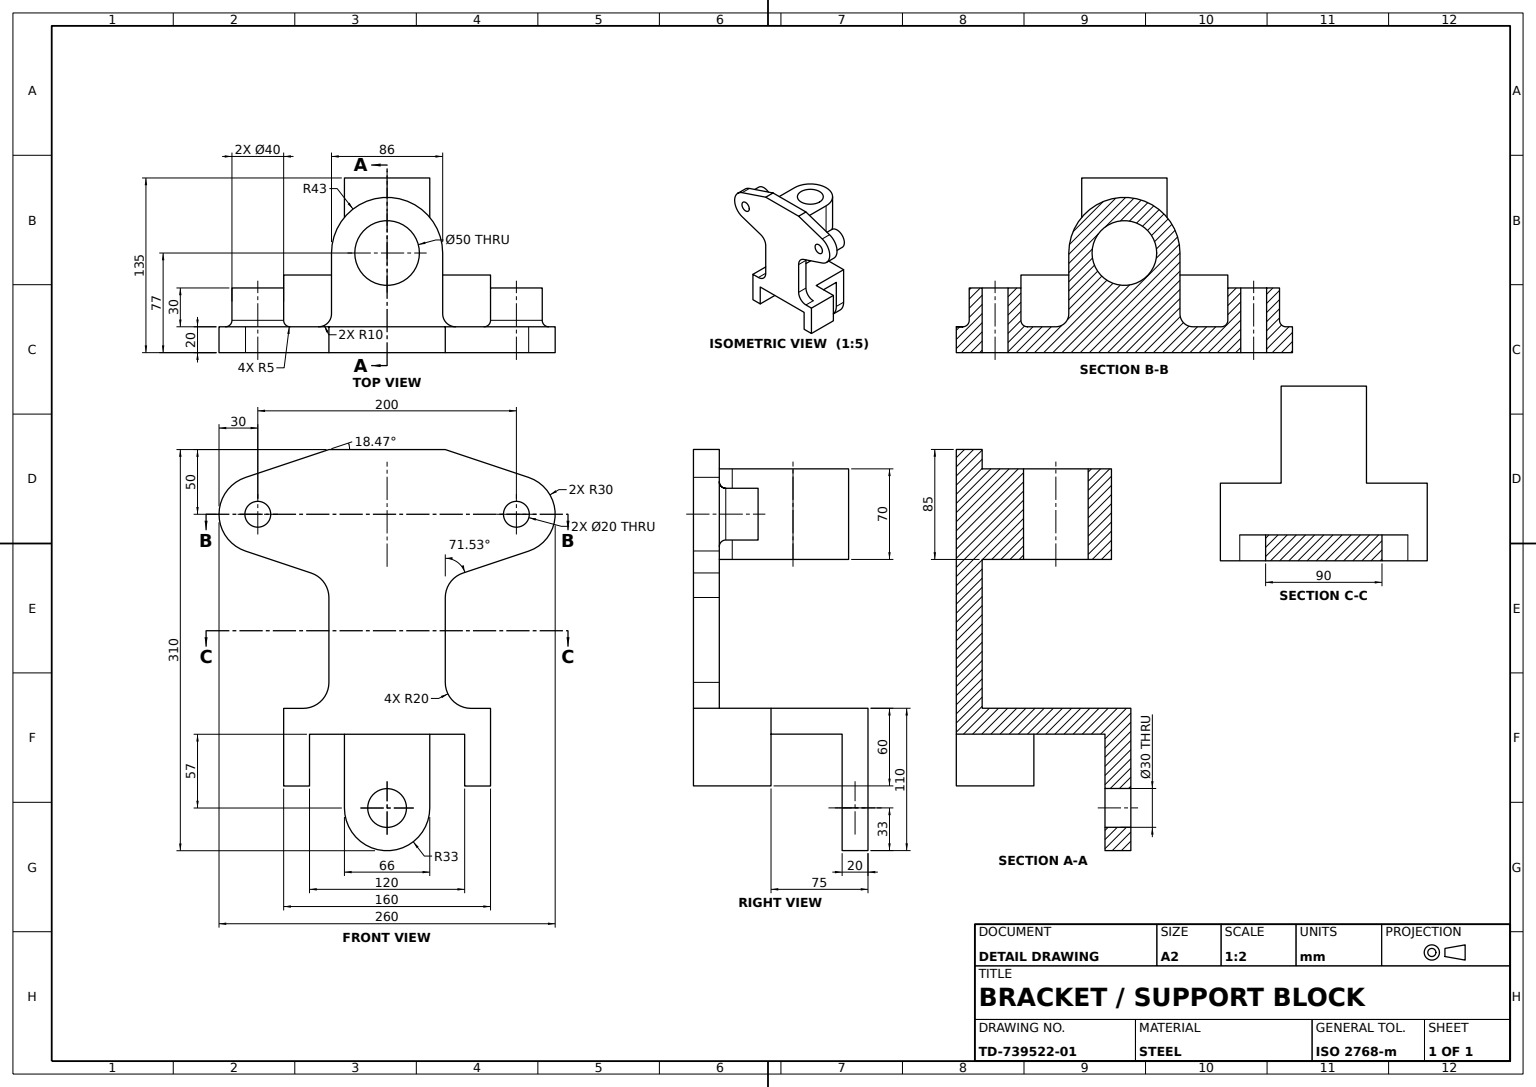
solid
v1 (-30,0,120)
v2 (-5,0,120)
e1 v1 v2 LINE
v3 (-30,0,80)
e2 v3 v1 CIRCLE(AX(P(-30,0,100),D(-1,0,0),D(0,0,-1)),20)
v4 (-5,0,80)
e3 v3 v4 LINE
e4 v4 v2 CIRCLE(AX(P(-5,0,100),D(-1,0,0),D(0,0,-1)),20)
face CYL(AX(P(-30,0,100),D(1,0,0),D(0,0,-1)),20) [-e1 -e2 e3 e4]
v5 (20,-130,-45)
v6 (20,-64.405882,-45)
e5 v5 v6 LINE
v7 (0,-130,-45)
e6 v5 v7 LINE
v8 (0,-64.405882,-45)
e7 v7 v8 LINE
e8 v6 v8 LINE
face PLANE(AX(P(20,-64.405882,-45),D(0,0,1),D(0,-1,0))) rev [-e5 e6 e7 -e8]
v9 (0,0,75)
v10 (0,0,125)
e9 v9 v10 CIRCLE(AX(P(0,0,100),D(1,0,0),D(0,0,-1)),25)
e10 v9 v4 CIRCLE(AX(P(-5,0,75),D(0,-1,0),D(0,0,-1)),5)
e11 v2 v4 CIRCLE(AX(P(-5,0,100),D(-1,0,0),D(0,0,-1)),20)
e12 v10 v2 CIRCLE(AX(P(-5,0,125),D(0,1,0),D(0,0,1)),5)
face TORUS(AX(P(-5,0,100),D(1,0,0),D(0,0,-1)),25,5) rev [-e9 e10 -e11 -e12]
v11 (0,-64.405882,45)
v12 (0,-130,45)
e13 v11 v12 LINE
v13 (20,-130,45)
e14 v12 v13 LINE
v14 (20,-64.405882,45)
e15 v14 v13 LINE
e16 v14 v11 LINE
face PLANE(AX(P(20,-64.405882,45),D(0,0,-1),D(0,1,0))) rev [e13 e14 -e15 e16]
v15 (20,-28.454684,109.504259)
v16 (20,-45.436092,58.663828)
e17 v15 v16 LINE
v17 (0,-28.454684,109.504259)
e18 v15 v17 LINE
v18 (0,-45.436092,58.663828)
e19 v17 v18 LINE
e20 v16 v18 LINE
face PLANE(AX(P(20,-45.436092,58.663828),D(0,0.948489482,-0.31680862),D(0,0.31680862,0.948489482))) rev [-e17 e18 e19 -e20]
v19 (-95,-170,-33)
v20 (-95,-227,-33)
e21 v19 v20 LINE
v21 (-95,-170,33)
e22 v19 v21 LINE
v22 (-95,-227,33)
e23 v22 v21 LINE
e24 v20 v22 CIRCLE(AX(P(-95,-227,0),D(-1,0,0),D(0,0,-1)),33)
v23 (-95,-227,15)
v24 (-95,-227,-15)
e25 v23 v24 CIRCLE(AX(P(-95,-227,0),D(-1,0,0),D(0,0,1)),15)
e26 v24 v23 CIRCLE(AX(P(-95,-227,0),D(-1,0,0),D(0,0,1)),15)
face PLANE(AX(P(-95,-227,0),D(1,0,0),D(0,0,-1))) [-e21 e22 -e23 -e24] [e25 e26]
v25 (-40,-150,-80)
v26 (20,-150,-80)
e27 v25 v26 LINE
v27 (20,-210,-80)
e28 v27 v26 LINE
v28 (-40,-210,-80)
e29 v28 v27 LINE
e30 v28 v25 LINE
face PLANE(AX(P(-40,-170,-80),D(0,0,1),D(1,0,0))) rev [e27 -e28 -e29 e30]
v29 (-115,-227,-33)
v30 (-115,-227,33)
e31 v29 v30 CIRCLE(AX(P(-115,-227,0),D(-1,0,0),D(0,0,-1)),33)
v31 (-115,-150,33)
e32 v30 v31 LINE
v32 (-115,-150,-33)
e33 v31 v32 LINE
e34 v29 v32 LINE
v33 (-115,-227,-15)
v34 (-115,-227,15)
e35 v33 v34 CIRCLE(AX(P(-115,-227,0),D(-1,0,0),D(0,0,1)),15)
e36 v34 v33 CIRCLE(AX(P(-115,-227,0),D(-1,0,0),D(0,0,1)),15)
face PLANE(AX(P(-115,-170,33),D(1,0,0),D(0,0,-1))) rev [e31 e32 e33 -e34] [-e35 -e36]
v35 (20,-45.436092,-58.663828)
e37 v6 v35 CIRCLE(AX(P(20,-64.405882,-65),D(-1,0,0),D(0,0,-1)),20)
v36 (0,-45.436092,-58.663828)
e38 v8 v36 CIRCLE(AX(P(0,-64.405882,-65),D(-1,0,0),D(0,0,-1)),20)
e39 v35 v36 LINE
face CYL(AX(P(20,-64.405882,-65),D(-1,0,0),D(0,0,1)),20) rev [-e37 e8 e38 -e39]
v37 (-40,-170,-60)
v38 (20,-170,-60)
e40 v37 v38 LINE
v39 (-40,-210,-60)
e41 v37 v39 LINE
v40 (20,-210,-60)
e42 v39 v40 LINE
e43 v40 v38 LINE
face PLANE(AX(P(0,0,-60),D(0,0,-1),D(1,0,0))) rev [-e40 e41 e42 e43]
v41 (20,0,90)
v42 (20,0,110)
e44 v41 v42 CIRCLE(AX(P(20,0,100),D(-1,0,0),D(0,0,1)),10)
v43 (-30,0,90)
e45 v41 v43 LINE
v44 (-30,0,110)
e46 v43 v44 CIRCLE(AX(P(-30,0,100),D(-1,0,0),D(0,0,1)),10)
e47 v42 v44 LINE
face CYL(AX(P(20,0,100),D(-1,0,0),D(0,0,1)),10) rev [-e44 e45 e46 -e47]
v45 (20,0,130)
v46 (0,0,130)
e48 v45 v46 LINE
v47 (20,28.454684,109.504259)
e49 v47 v45 CIRCLE(AX(P(20,0,100),D(1,0,0),D(0,0,-1)),30)
v48 (0,28.454684,109.504259)
e50 v47 v48 LINE
e51 v48 v46 CIRCLE(AX(P(0,0,100),D(1,0,0),D(0,0,-1)),30)
face CYL(AX(P(20,0,100),D(-1,0,0),D(0,0,1)),30) [-e48 -e49 e50 e51]
e52 v10 v9 CIRCLE(AX(P(0,0,100),D(1,0,0),D(0,0,-1)),25)
face TORUS(AX(P(-5,0,100),D(1,0,0),D(0,0,-1)),25,5) rev [e12 -e4 -e10 -e52]
e53 v46 v17 CIRCLE(AX(P(0,0,100),D(1,0,0),D(0,0,-1)),30)
e54 v45 v15 CIRCLE(AX(P(20,0,100),D(1,0,0),D(0,0,-1)),30)
face CYL(AX(P(20,0,100),D(-1,0,0),D(0,0,1)),30) [e53 -e18 -e54 e48]
e55 v40 v27 LINE
v49 (20,-150,-65)
e56 v26 v49 LINE
e57 v49 v5 CIRCLE(AX(P(20,-130,-65),D(-1,0,0),D(0,0,-1)),20)
v50 (20,-28.454684,-109.504259)
e58 v35 v50 LINE
v51 (20,28.454684,-109.504259)
e59 v50 v51 CIRCLE(AX(P(20,0,-100),D(1,0,0),D(0,0,-1)),30)
v52 (20,50,-45)
e60 v51 v52 LINE
v53 (20,50,45)
e61 v52 v53 LINE
e62 v53 v47 LINE
e63 v16 v14 CIRCLE(AX(P(20,-64.405882,65),D(-1,0,0),D(0,0,1)),20)
v54 (20,-150,65)
e64 v13 v54 CIRCLE(AX(P(20,-130,65),D(-1,0,0),D(0,0,-1)),20)
v55 (20,-150,80)
e65 v54 v55 LINE
v56 (20,-210,80)
e66 v56 v55 LINE
v57 (20,-210,60)
e67 v57 v56 LINE
v58 (20,-170,60)
e68 v57 v58 LINE
e69 v38 v58 LINE
v59 (20,0,-110)
v60 (20,0,-90)
e70 v59 v60 CIRCLE(AX(P(20,0,-100),D(-1,0,0),D(0,0,1)),10)
e71 v60 v59 CIRCLE(AX(P(20,0,-100),D(-1,0,0),D(0,0,1)),10)
e72 v42 v41 CIRCLE(AX(P(20,0,100),D(-1,0,0),D(0,0,1)),10)
face PLANE(AX(P(20,0,-100),D(1,0,0),D(0,0,-1))) [-e43 e55 e28 e56 e57 e5 e37 e58 e59 e60 e61 e62 e49 e54 e17 e63 e15 e64 e65 -e66 -e67 e68 -e69] [e70 e71] [e44 e72]
v61 (-40,-210,80)
v62 (-40,-150,80)
e73 v61 v62 LINE
e74 v61 v56 LINE
e75 v55 v62 LINE
face PLANE(AX(P(20,-170,80),D(0,0,-1),D(-1,0,0))) rev [-e73 e74 e66 e75]
v63 (-40,-150,33)
e76 v63 v31 LINE
e77 v62 v63 LINE
v64 (0,-150,65)
e78 v54 v64 LINE
v65 (0,-150,-65)
e79 v64 v65 LINE
e80 v65 v49 LINE
v66 (-40,-150,-33)
e81 v66 v25 LINE
e82 v32 v66 LINE
face PLANE(AX(P(0,-150,0),D(0,-1,0),D(0,0,-1))) rev [-e33 -e76 -e77 -e75 -e65 e78 e79 e80 -e56 -e27 -e81 -e82]
v67 (-57,35,-43)
v68 (-57,35,43)
e83 v67 v68 CIRCLE(AX(P(-57,35,0),D(0,1,0),D(0,0,1)),43)
v69 (-57,-35,-43)
e84 v67 v69 LINE
v70 (-57,-35,43)
e85 v69 v70 CIRCLE(AX(P(-57,-35,0),D(0,1,0),D(0,0,1)),43)
e86 v68 v70 LINE
face CYL(AX(P(-57,35,0),D(0,-1,0),D(0,0,-1)),43) [-e83 e84 e85 -e86]
v71 (-5,0,-80)
v72 (-5,0,-120)
e87 v71 v72 CIRCLE(AX(P(-5,0,-100),D(-1,0,0),D(0,0,-1)),20)
v73 (-30,0,-120)
e88 v73 v72 LINE
v74 (-30,0,-80)
e89 v74 v73 CIRCLE(AX(P(-30,0,-100),D(-1,0,0),D(0,0,1)),20)
e90 v74 v71 LINE
face CYL(AX(P(-30,0,-100),D(1,0,0),D(0,0,-1)),20) [e87 -e88 -e89 e90]
v75 (-10,35,-43)
e91 v75 v67 LINE
v76 (-10,-35,-43)
e92 v75 v76 LINE
e93 v76 v69 LINE
face PLANE(AX(P(-57,35,-43),D(0,0,1),D(1,0,0))) rev [-e84 -e91 e92 e93]
v77 (-57,35,-25)
v78 (-57,35,25)
e94 v77 v78 CIRCLE(AX(P(-57,35,0),D(0,1,0),D(0,0,1)),25)
e95 v78 v77 CIRCLE(AX(P(-57,35,0),D(0,1,0),D(0,0,1)),25)
v79 (0,35,-53)
e96 v79 v75 CIRCLE(AX(P(-10,35,-53),D(0,-1,0),D(0,0,1)),10)
v80 (-10,35,43)
e97 v68 v80 LINE
v81 (0,35,53)
e98 v80 v81 CIRCLE(AX(P(-10,35,53),D(0,-1,0),D(0,0,1)),10)
e99 v81 v79 LINE
face PLANE(AX(P(-57,35,0),D(0,1,0),D(0,0,1))) [-e94 -e95] [e96 e91 e83 e97 e98 e99]
e100 v20 v29 LINE
v82 (-40,-170,-33)
e101 v82 v66 LINE
e102 v19 v82 LINE
face PLANE(AX(P(-115,-170,-33),D(0,0,1),D(1,0,0))) rev [e100 e34 e82 -e101 -e102 e21]
e103 v22 v30 LINE
v83 (-40,-170,33)
e104 v83 v21 LINE
e105 v83 v63 LINE
face PLANE(AX(P(-40,-170,33),D(0,0,-1),D(-1,0,0))) rev [e76 -e32 -e103 e23 -e104 e105]
v84 (0,0,-125)
e106 v84 v72 CIRCLE(AX(P(-5,0,-125),D(0,-1,0),D(0,0,-1)),5)
v85 (0,0,-75)
e107 v85 v71 CIRCLE(AX(P(-5,0,-75),D(0,1,0),D(0,0,1)),5)
e108 v84 v85 CIRCLE(AX(P(0,0,-100),D(1,0,0),D(0,0,-1)),25)
face TORUS(AX(P(-5,0,-100),D(1,0,0),D(0,0,-1)),25,5) rev [e106 -e87 -e107 -e108]
v86 (0,-28.454684,-109.504259)
e109 v36 v86 LINE
e110 v50 v86 LINE
face PLANE(AX(P(20,-28.454684,-109.504259),D(0,0.948489482,0.31680862),D(0,-0.31680862,0.948489482))) rev [-e58 e39 e109 -e110]
face CYL(AX(P(-95,-227,0),D(-1,0,0),D(0,0,1)),33) [-e31 -e100 e24 e103]
v87 (0,-35,53)
v88 (-10,-35,43)
e111 v87 v88 CIRCLE(AX(P(-10,-35,53),D(0,1,0),D(0,0,1)),10)
e112 v81 v87 LINE
e113 v88 v80 LINE
face CYL(AX(P(-10,0,53),D(0,1,0),D(0,0,1)),10) rev [-e111 -e112 -e98 -e113]
v89 (-40,-170,60)
e114 v58 v89 LINE
v90 (-40,-210,60)
e115 v90 v57 LINE
e116 v89 v90 LINE
face PLANE(AX(P(0,0,60),D(0,0,1),D(1,0,0))) rev [-e114 -e68 -e115 -e116]
v91 (-30,0,-90)
v92 (-30,0,-110)
e117 v91 v92 CIRCLE(AX(P(-30,0,-100),D(-1,0,0),D(0,0,1)),10)
e118 v59 v92 LINE
e119 v60 v91 LINE
face CYL(AX(P(20,0,-100),D(-1,0,0),D(0,0,1)),10) rev [e117 -e118 -e71 e119]
e120 v39 v28 LINE
face PLANE(AX(P(-40,-210,-60),D(0,1,0),D(0,0,1))) rev [e120 e29 -e55 -e42]
v93 (0,28.454684,-109.504259)
e121 v51 v93 LINE
v94 (0,50,-45)
e122 v93 v94 LINE
e123 v52 v94 LINE
face PLANE(AX(P(20,28.454684,-109.504259),D(0,-0.948489482,0.31680862),D(0,-0.31680862,-0.948489482))) rev [-e60 e121 e122 -e123]
e124 v7 v65 CIRCLE(AX(P(0,-130,-65),D(1,0,0),D(0,0,-1)),20)
e125 v64 v12 CIRCLE(AX(P(0,-130,65),D(1,0,0),D(0,0,-1)),20)
e126 v18 v11 CIRCLE(AX(P(0,-64.405882,65),D(-1,0,0),D(0,0,1)),20)
v95 (0,50,45)
e127 v95 v48 LINE
e128 v94 v95 LINE
e129 v86 v93 CIRCLE(AX(P(0,0,-100),D(1,0,0),D(0,0,-1)),30)
e130 v85 v84 CIRCLE(AX(P(0,0,-100),D(1,0,0),D(0,0,-1)),25)
v96 (0,-35,-53)
e131 v96 v79 LINE
e132 v87 v96 LINE
face PLANE(AX(P(0,0,-100),D(1,0,0),D(0,0,-1))) rev [e9 e52] [e124 -e79 e125 -e13 -e126 -e19 -e53 -e51 -e127 -e128 -e122 -e129 -e109 -e38 -e7] [e108 e130] [e131 -e99 e112 e132]
e133 v72 v71 CIRCLE(AX(P(-5,0,-100),D(-1,0,0),D(0,0,-1)),20)
face TORUS(AX(P(-5,0,-100),D(1,0,0),D(0,0,-1)),25,5) rev [-e133 -e106 -e130 e107]
e134 v53 v95 LINE
face PLANE(AX(P(20,50,-45),D(0,-1,0),D(0,0,-1))) rev [-e61 e123 e128 -e134]
e135 v82 v37 LINE
e136 v89 v83 LINE
face PLANE(AX(P(0,-170,0),D(0,-1,0),D(0,0,-1))) [e104 -e22 e102 e135 e40 e69 e114 e136]
e137 v90 v61 LINE
face PLANE(AX(P(-40,-210,60),D(0,-1,0),D(0,0,-1))) [-e74 -e137 e115 e67]
e138 v70 v88 LINE
face PLANE(AX(P(0,35,43),D(0,0,-1),D(-1,0,0))) rev [-e97 e86 e138 e113]
v97 (-57,-35,25)
e139 v78 v97 LINE
v98 (-57,-35,-25)
e140 v98 v97 CIRCLE(AX(P(-57,-35,0),D(0,1,0),D(0,0,1)),25)
e141 v77 v98 LINE
face CYL(AX(P(-57,35,0),D(0,-1,0),D(0,0,-1)),25) rev [e139 -e140 -e141 e94]
e142 v44 v43 CIRCLE(AX(P(-30,0,100),D(-1,0,0),D(0,0,1)),10)
face CYL(AX(P(20,0,100),D(-1,0,0),D(0,0,1)),10) rev [-e72 e47 e142 -e45]
e143 v92 v91 CIRCLE(AX(P(-30,0,-100),D(-1,0,0),D(0,0,1)),10)
face CYL(AX(P(20,0,-100),D(-1,0,0),D(0,0,1)),10) rev [-e119 -e70 e118 e143]
e144 v23 v34 LINE
e145 v24 v33 LINE
face CYL(AX(P(-95,-227,0),D(-1,0,0),D(0,0,1)),15) rev [e35 -e144 -e26 e145]
face PLANE(AX(P(-40,-170,80),D(1,0,0),D(0,0,-1))) rev [e137 e73 e77 -e105 -e136 e116]
face PLANE(AX(P(20,50,45),D(0,-0.948489482,-0.31680862),D(0,0.31680862,-0.948489482))) rev [-e62 e134 e127 -e50]
face PLANE(AX(P(-40,-170,-33),D(1,0,0),D(0,0,-1))) rev [-e30 -e120 -e41 -e135 e101 e81]
e146 v97 v98 CIRCLE(AX(P(-57,-35,0),D(0,1,0),D(0,0,1)),25)
face CYL(AX(P(-57,35,0),D(0,-1,0),D(0,0,-1)),25) rev [-e146 -e139 e95 e141]
e147 v76 v96 CIRCLE(AX(P(-10,-35,-53),D(0,1,0),D(0,0,1)),10)
face CYL(AX(P(-10,35,-53),D(0,1,0),D(0,0,1)),10) rev [-e96 -e131 -e147 -e92]
e148 v1 v3 CIRCLE(AX(P(-30,0,100),D(-1,0,0),D(0,0,-1)),20)
face CYL(AX(P(-30,0,100),D(1,0,0),D(0,0,-1)),20) [e11 -e3 -e148 e1]
face CYL(AX(P(20,0,-100),D(-1,0,0),D(0,0,1)),30) [-e59 e110 e129 -e121]
face CYL(AX(P(0,-130,65),D(1,0,0),D(0,0,-1)),20) rev [-e78 -e64 -e14 -e125]
face CYL(AX(P(20,-64.405882,65),D(-1,0,0),D(0,0,1)),20) rev [e20 e126 -e16 -e63]
e149 v73 v74 CIRCLE(AX(P(-30,0,-100),D(-1,0,0),D(0,0,1)),20)
face PLANE(AX(P(-30,0,-100),D(-1,0,0),D(0,0,1))) [-e117 -e143] [e149 e89]
face PLANE(AX(P(-57,-35,0),D(0,1,0),D(0,0,1))) rev [e146 e140] [-e85 -e93 e147 -e132 e111 -e138]
face CYL(AX(P(-95,-227,0),D(-1,0,0),D(0,0,1)),15) rev [-e25 e144 e36 -e145]
face CYL(AX(P(20,-130,-65),D(1,0,0),D(0,0,-1)),20) rev [-e124 -e6 -e57 -e80]
face PLANE(AX(P(-30,0,100),D(1,0,0),D(0,0,-1))) rev [-e46 -e142] [e148 e2]
face CYL(AX(P(-30,0,-100),D(1,0,0),D(0,0,-1)),20) [e88 e133 -e90 -e149]
